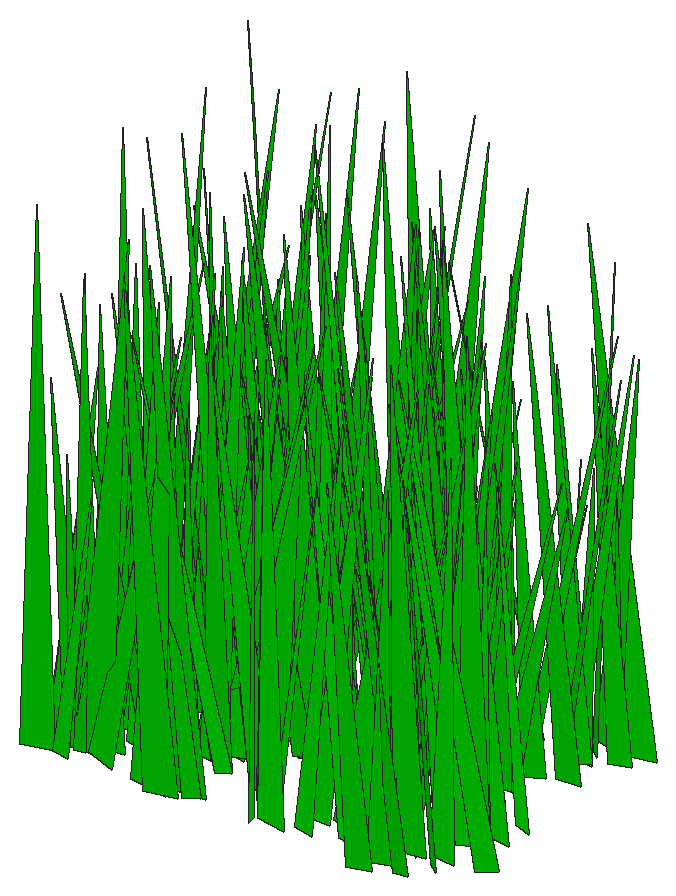
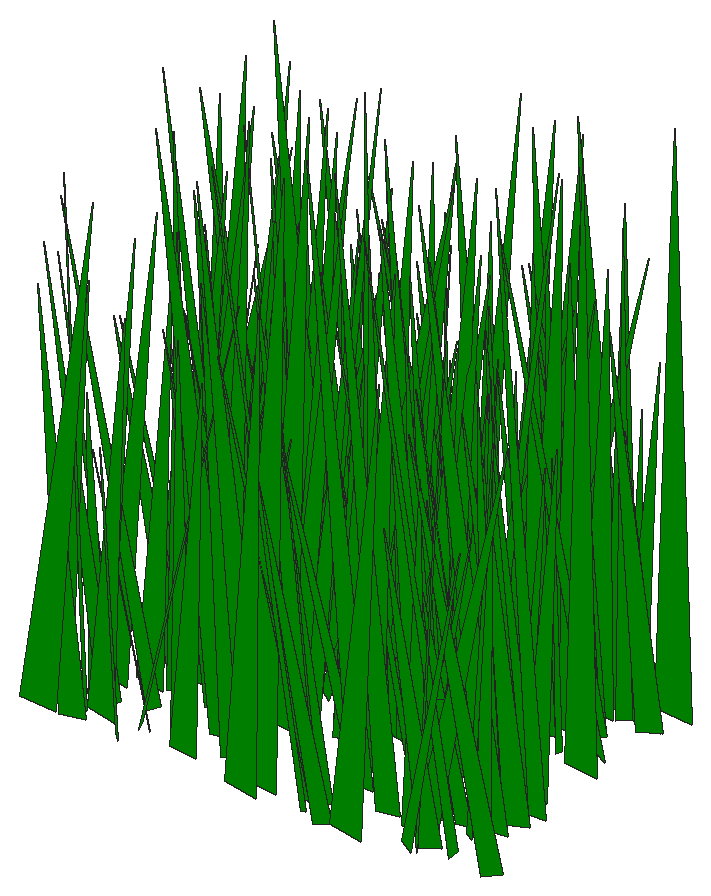
# SketchUp Ruby script. Lengths in inches.
U = 1.inch
M = Sketchup.active_model
def pt(a) = Geom::Point3d.new(a.map { |v| v * U })
def face(e, loops, mat)
  f = e.add_face(loops[0].map { |a| pt(a) })
  loops[1..].each { |l| e.add_face(l.map { |a| pt(a) }).erase! }
  f.material = f.back_material = mat if mat
  f
end
# faces: each face lists its corners as indices into pts; further lists are holes
def faces(e, pts, list, mat = nil) = list.each { |f| face(e, (f[0].is_a?(Array) ? f : [f]).map { |l| l.map { |i| pts[i] } }, mat) }
# xy, xz, yz: faces in a plane at the given z, y or x. An outline is a flat list of corners, or four numbers for a rectangle; further outlines are holes
def ring(l) = l.size == 4 ? [[l[0], l[1]], [l[2], l[1]], [l[2], l[3]], [l[0], l[3]]] : l.each_slice(2).to_a
def flat(e, list, mat, &to3) = list.each { |f| face(e, (f[0].is_a?(Array) ? f : [f]).map { |l| ring(l).map { |u, v| to3.(u, v) } }, mat) }
def xy(e, z, list, mat = nil) = flat(e, list, mat) { |x, y| [x, y, z] }
def xz(e, y, list, mat = nil) = flat(e, list, mat) { |x, z| [x, y, z] }
def yz(e, x, list, mat = nil) = flat(e, list, mat) { |y, z| [x, y, z] }
def lines(e, pts, list) = list.each { |a, b| e.add_line(pt(pts[a]), pt(pts[b])) }
# prism: a flat outline (further loops are holes) pulled along v
def prism(e, loops, v, mat = nil)
  f = face(e, loops, mat); d = Geom::Vector3d.new(v.map { |x| x * U })
  f.pushpull(f.normal.samedirection?(d) ? d.length : -d.length)
end
def box(e, o, s, mat = nil) = prism(e, [[o, [o[0] + s[0], o[1], o[2]], [o[0] + s[0], o[1] + s[1], o[2]], [o[0], o[1] + s[1], o[2]]]], [0, 0, s[2]], mat)
def at(x, y, z, deg = 0) = Geom::Transformation.translation(pt([x, y, z])) * Geom::Transformation.rotation(ORIGIN, Z_AXIS, deg.degrees)
def axes(o, x, y, z) = Geom::Transformation.new([*x, 0, *y, 0, *z, 0, *pt(o).to_a, 1])
def part(name) = M.definitions.add(name)
# library, detail: a bought-in or finely detailed component or shape, given as its bounding box
def library(name, o, s) = part(name).tap { |d| box(d.entities, o, s) }
def detail(e, o, s) = box(e.add_group.entities, o, s)
def put(e, d, t, mat = nil) = e.add_instance(d, t).tap { |i| i.material = mat if mat }
def group(e, t, mat = nil) = e.add_group.tap { |g| g.transformation = t; g.material = mat if mat }.entities
root = M.entities
M.materials.add("[Color G06]").color = [0, 204, 0]
c1 = part("fur_instance\#9")
p = [[0.8125,0,1.79],[0.67,-0.02,1.48],[0,-0.11,0],[0,0.11,0]]
faces(c1.entities,p,[[0,1,2,3]])
put(root,c1,axes([54.39,21.29,4.28],[-0.32887,0.46438,1.72986],[3.51347,0.02974,0.5749],[-0.29205,-0.16513,4.96826]),"[Color G06]")
put(root,c1,axes([54.4,23.9,4.28],[4.17535,-0.0739,3.413],[-0.23891,-0.66047,-0.99003],[-2.33208,-0.06466,6.21204]),"[Color G06]")
put(root,c1,axes([55.41,24.38,4.28],[-3.216,0.412,0.55463],[2.97627,0.4423,0.80624],[-0.09509,-0.09034,6.47707]),"[Color G06]")
put(root,c1,axes([54.22,23.56,4.28],[3.35775,0.35388,2.56454],[2.52243,-0.52084,0.8788],[-1.73834,-0.07222,6.2288]),"[Color G06]")
put(root,c1,axes([52.72,25.09,4.28],[3.14492,-0.38862,0.66664],[-2.81983,-0.42872,1.00531],[0.11909,0.11131,6.19928]),"[Color G06]")
put(root,c1,axes([54.25,15.9,4.28],[2.70284,-0.68709,2.07562],[-4.99876,-0.40147,-0.72645],[-1.10438,0.13558,8.36796]),"[Color G06]")
put(root,c1,axes([53.69,22.07,4.28],[4.95219,0.39046,2.95138],[3.0826,-0.719,-0.62677],[-1.49582,-0.18905,8.47946]),"[Color G06]")
put(root,c1,axes([54.32,19.52,4.28],[3.96209,-0.57788,2.65528],[-4.16866,-0.59516,-0.98497],[-1.71829,0.1114,8.51222]),"[Color G06]")
put(root,c1,axes([54.9,16.7,4.28],[0.16857,0.49558,1.55991],[3.65308,-0.04633,0.80895],[-0.61231,-0.13996,5.25573]),"[Color G06]")
put(root,c1,axes([55.3125,25.28,4.28],[-2.75872,-0.20781,0.94511],[-1.59434,0.37899,-0.8224],[0.28094,0.11013,4.61354]),"[Color G06]")
put(root,c1,axes([54.84,21.24,4.28],[2.06181,0.28515,2.25548],[2.13746,-0.34115,0.59003],[-1.37485,-0.10276,4.29978]),"[Color G06]")
put(root,c1,axes([55.1,25.16,4.28],[-5.73799,-0.08046,2.98882],[-0.8058,0.83989,-0.85823],[1.91905,0.11209,8.57626]),"[Color G06]")
put(root,c1,axes([53.79,22.75,4.28],[0.61886,-0.50723,0.31793],[-3.60857,-0.08115,0.81733],[0.50473,0.04173,5.45369]),"[Color G06]")
put(root,c1,axes([54.17,16.89,4.28],[0.36145,-0.35493,1.94549],[-2.84398,-0.026,0.63535],[0.29127,0.18658,3.78944]),"[Color G06]")
put(root,c1,axes([54.19,16.95,4.28],[-0.4395,0.54622,1.08378],[3.90573,0.07911,-1.04214],[0.78414,-0.08788,5.79824]),"[Color G06]")
put(root,c1,axes([54.52,22.86,4.28],[-1.83901,-0.44209,2.47492],[-3.40475,0.29592,0.42094],[1.09577,0.17753,5.46154]),"[Color G06]")
put(root,c1,axes([54.1,21.81,4.28],[3.61401,-0.17304,1.5239],[-1.34844,-0.5171,0.3982],[-0.87246,0.08243,5.69704]),"[Color G06]")
put(root,c1,axes([54.95,16.67,4.28],[-1.53114,-0.37036,0.85419],[-2.64416,0.22416,0.57766],[0.62379,0.04111,4.54534]),"[Color G06]")
put(root,c1,axes([53.98,22.42,4.28],[2.19139,-0.2507,0.50243],[-1.8224,-0.29307,0.9561],[0.15541,0.09841,4.1271]),"[Color G06]")
put(root,c1,axes([55.09,16.83,4.28],[4.06238,-0.21355,3.19268],[-1.8501,-0.62183,0.48051],[-1.86698,0.15154,6.4708]),"[Color G06]")
put(root,c1,axes([54.04,23.36,4.28],[3.9698,0.60491,1.9926],[4.50643,-0.55462,-0.71321],[-0.53613,-0.18276,8.75945]),"[Color G06]")
put(root,c1,axes([55.6,24.62,4.28],[0.92736,0.51655,0.50005],[3.6541,-0.1355,0.94194],[-0.69385,-0.02321,5.62895]),"[Color G06]")
put(root,c1,axes([54.64,21.84,4.28],[1.4992,0.48907,0.74233],[3.53969,-0.20399,-0.52959],[0.13419,-0.083,5.67598]),"[Color G06]")
put(root,c1,axes([55.26,16.42,4.28],[2.49706,0.29446,1.60599],[2.14462,-0.37344,0.41704],[-1.00716,-0.06513,4.86978]),"[Color G06]")
put(root,c1,axes([54.79,24.99,4.28],[-0.05361,0.4756,0.01399],[3.34161,0.00759,-1.02035],[0.68277,0.00022,4.99493]),"[Color G06]")
put(root,c1,axes([56.28,23.64,4.28],[-2.08549,-0.28281,0.67775],[-2.07819,0.2842,-0.66105],[0.00923,0.08832,4.29725]),"[Color G06]")
put(root,c1,axes([55.39,16.55,4.28],[1.69023,-0.63644,1.78454],[-4.66449,-0.25194,-0.45308],[-0.70656,0.14072,7.26]),"[Color G06]")
put(root,c1,axes([55.33,19.16,4.28],[2.45742,0.11817,1.80132],[1.13854,-0.35975,-0.75845],[-0.93512,-0.12747,3.81028]),"[Color G06]")
put(root,c1,axes([55.16,17.59,4.28],[2.74488,-0.06523,1.24442],[-0.40367,-0.39945,-0.41655],[-0.86554,-0.02058,4.14068]),"[Color G06]")
put(root,c1,axes([54.98,15.96,4.28],[1.92096,-0.27343,1.19339],[-2.10067,-0.26489,0.58119],[-0.26385,0.11826,4.06121]),"[Color G06]")
put(root,c1,axes([54.13,24.88,4.28],[5.77126,-0.07264,1.65356],[-0.6218,-0.81519,0.73366],[-1.05301,0.08323,8.62952]),"[Color G06]")
put(root,c1,axes([55.86,16.97,4.28],[-0.07198,0.64257,1.00658],[4.64555,0.00333,0.49762],[-0.32595,-0.09439,6.86985]),"[Color G06]")
put(root,c1,axes([55.76,18.18,4.28],[0.38893,0.70323,0.41389],[5.03381,-0.05713,0.58507],[-0.41212,-0.03418,7.53692]),"[Color G06]")
put(root,c1,axes([55.11,21.39,4.28],[-2.85975,0.29525,3.99207],[2.87232,0.47051,0.59866],[1.83502,-0.27635,5.28429]),"[Color G06]")
put(root,c1,axes([54.86,23.54,4.28],[1.90639,0.3389,0.36117],[2.44012,-0.26248,-0.47701],[0.10354,-0.05392,4.59177]),"[Color G06]")
put(root,c1,axes([54.96,22.7,4.28],[-2.44366,-0.51435,4.27043],[-4.22034,0.43545,0.6304],[1.98946,0.29197,6.58268]),"[Color G06]")
put(root,c1,axes([56.14,23.07,4.28],[-2.4222,-0.16072,1.56561],[-1.40113,0.3428,-0.79952],[0.68014,0.13382,3.92857]),"[Color G06]")
put(root,c1,axes([56.84,18.28,4.28],[2.06357,-0.41111,4.06457],[-3.41801,-0.4034,-0.81078],[-2.09874,0.25276,5.3169]),"[Color G06]")
put(root,c1,axes([55.32,17.73,4.28],[2.4105,-0.28915,0.19332],[-2.00695,-0.33122,-1.01055],[-0.53712,-0.06004,4.64352]),"[Color G06]")
put(root,c1,axes([57.46,16.8,4.28],[-3.99959,-0.37213,0.86302],[-2.72854,0.55002,-1.00142],[0.10108,0.12253,7.11603]),"[Color G06]")
put(root,c1,axes([54.55,18.6,4.28],[4.47178,0.41149,0.17523],[2.91592,-0.6199,1.00676],[-0.46818,0.06949,7.94392]),"[Color G06]")
put(root,c1,axes([57.03,20.02,4.28],[-5.43427,-0.32024,1.64444],[-2.20505,0.77263,1.00717],[1.2737,-0.02872,8.75967]),"[Color G06]")
put(root,c1,axes([56.06,19.92,4.28],[-1.94851,-0.34259,1.45943],[-2.44364,0.29794,0.74664],[1.00898,0.05999,4.62667]),"[Color G06]")
put(root,c1,axes([56.49,18.41,4.28],[1.89484,-0.65521,2.90311],[-4.94694,-0.30434,-0.67805],[-1.17417,0.22486,7.54167]),"[Color G06]")
put(root,c1,axes([55.21,20.34,4.28],[2.42337,0.26843,0.58382],[1.96182,-0.32647,-0.94651],[0.09764,-0.10286,4.52767]),"[Color G06]")
put(root,c1,axes([55.08,17.96,4.28],[3.47494,-0.38303,1.16165],[-2.84618,-0.47804,0.91113],[-0.22013,0.13428,6.55718]),"[Color G06]")
put(root,c1,axes([55.64,16.5,4.28],[1.06191,-0.77881,1.43715],[-5.65566,-0.13692,0.81096],[0.36184,0.14546,8.45802]),"[Color G06]")
put(root,c1,axes([56.25,20.77,4.28],[-0.48812,-0.56435,0.59145],[-4.0461,0.07295,0.53768],[0.40605,0.04854,6.06878]),"[Color G06]")
put(root,c1,axes([56.42,17.59,4.28],[-0.81081,0.43637,0.59606],[3.1308,0.11836,-0.44094],[0.38738,-0.04321,4.81134]),"[Color G06]")
put(root,c1,axes([55.9,19.44,4.28],[-2.00864,0.36267,2.32372],[2.62384,0.33828,-0.99869],[1.51554,-0.105,4.80878]),"[Color G06]")
put(root,c1,axes([56.95,25.68,4.28],[0.02737,-0.60684,1.90999],[-4.50307,-0.02493,-0.76568],[-0.54191,0.17649,6.45898]),"[Color G06]")
put(root,c1,axes([55.82,23.73,4.28],[2.15587,0.69515,2.44048],[5.24335,-0.29297,-0.76006],[-0.15789,-0.23747,8.08183]),"[Color G06]")
put(root,c1,axes([56.49,17.54,4.28],[-1.58986,0.63127,0.88104],[4.48752,0.23209,-1.01454],[0.83865,-0.04518,7.09892]),"[Color G06]")
put(root,c1,axes([55.61,22.13,4.28],[3.80806,0.03495,0.96703],[0.35187,-0.53107,-0.89046],[-0.59803,-0.08994,5.6338]),"[Color G06]")
put(root,c1,axes([56.38,18.66,4.28],[-0.3077,-0.67019,0.64192],[-4.80571,0.04796,0.60615],[0.43369,0.05593,7.17218]),"[Color G06]")
put(root,c1,axes([56.35,22.41,4.28],[2.4729,0.11645,1.4233],[1.02559,-0.35504,-0.64338],[-0.74329,-0.10245,3.84757]),"[Color G06]")
put(root,c1,axes([56.45,20.07,4.28],[2.32899,-0.5225,0.84399],[-3.72888,-0.33246,-0.65873],[-0.674,0.03384,6.5608]),"[Color G06]")
put(root,c1,axes([57.51,21.8,4.28],[-0.5988,0.63341,0.59432],[4.53264,0.0766,0.82237],[-0.49597,-0.06464,6.798]),"[Color G06]")
put(root,c1,axes([57.01,18.22,4.28],[1.53188,0.34391,1.42378],[2.4933,-0.23899,0.6392],[-0.87952,-0.0785,4.29188]),"[Color G06]")
put(root,c1,axes([56.7,21.53,4.28],[2.75815,-0.30181,0.88619],[-2.08377,-0.39307,-0.89114],[-0.83298,-0.01604,5.16358]),"[Color G06]")
put(root,c1,axes([56.01,16.37,4.28],[2.13686,0.51171,0.80614],[3.69412,-0.28584,-1.02976],[0.33236,-0.11287,6.26251]),"[Color G06]")
put(root,c1,axes([58.96,17.89,4.28],[-3.87655,0.3039,0.26995],[2.18653,0.53782,0.58576],[-0.03539,-0.05997,6.62074]),"[Color G06]")
put(root,c1,axes([57.57,18.24,4.28],[1.99902,0.36205,1.56743],[2.5928,-0.30718,0.76441],[-1.05747,-0.06877,4.83731]),"[Color G06]")
put(root,c1,axes([56.73,24.25,4.28],[4.51231,0.50928,2.87399],[3.98181,-0.64173,-0.90131],[-1.08694,-0.23665,8.62924]),"[Color G06]")
put(root,c1,axes([57.11,21.39,4.28],[2.71803,-0.17288,1.5082],[-1.45728,-0.38206,0.83558],[-0.65701,0.13223,4.38604]),"[Color G06]")
put(root,c1,axes([57.37,20.51,4.28],[3.59461,-0.15483,2.07327],[-1.27584,-0.52874,0.40506],[-1.23671,0.09543,5.60827]),"[Color G06]")
put(root,c1,axes([58.6,18.72,4.28],[-5.08907,0.45043,2.63466],[3.43381,0.7321,0.43775],[1.32304,-0.1675,8.99813]),"[Color G06]")
put(root,c1,axes([57.23,21.55,4.28],[3.53384,-0.42545,1.3267],[-3.03521,-0.50675,-0.60886],[-0.94033,0.03682,6.95111]),"[Color G06]")
put(root,c1,axes([58.39,15.9375,4.28],[0.15133,-0.73593,1.78238],[-5.37361,-0.03986,-0.87169],[-0.63166,0.16282,7.84263]),"[Color G06]")
put(root,c1,axes([57.79,21.41,4.28],[-1.28026,0.55064,0.96088],[3.92353,0.19121,-0.91038],[0.78247,-0.05785,6.13705]),"[Color G06]")
put(root,c1,axes([58.72,22.66,4.28],[-0.92109,0.66321,2.02919],[4.94228,0.11589,0.65999],[-0.19317,-0.19726,7.21021]),"[Color G06]")
put(root,c1,axes([57.92,16.02,4.28],[-0.71518,0.71953,2.07998],[5.30775,0.11849,-0.6322],[0.62412,-0.18321,7.75991]),"[Color G06]")
put(root,c1,axes([58.87,19.34,4.28],[1.63729,0.51899,3.33742],[4.11223,-0.29196,0.70908],[-1.38849,-0.25268,6.03548]),"[Color G06]")
put(root,c1,axes([57.82,18.43,4.28],[2.12451,0.36732,0.0027],[2.61968,-0.29466,0.52674],[-0.27546,0.03066,5.03029]),"[Color G06]")
put(root,c1,axes([59.17,19.12,4.28],[-1.39523,0.73043,1.61988],[5.3465,0.18562,0.6715],[-0.16474,-0.16199,8.07378]),"[Color G06]")
put(root,c1,axes([58.95,16.4,4.28],[-0.78502,-0.76352,1.32542],[-5.54355,0.10374,-0.46905],[-0.18897,0.1285,8.25378]),"[Color G06]")
put(root,c1,axes([59.21,21.04,4.28],[-2.102,0.46139,1.74394],[3.50405,0.28558,0.75485],[0.17569,-0.1756,5.80984]),"[Color G06]")
put(root,c1,axes([57.59,19.98,4.28],[3.03483,-0.40436,0.19445],[-2.88553,-0.42312,-0.47865],[-0.31514,-0.01981,6.25516]),"[Color G06]")
put(root,c1,axes([59.16,16.29,4.28],[0.79739,-0.36655,2.11193],[-2.80611,-0.16152,-0.85385],[-1.01602,0.15843,4.01571]),"[Color G06]")
put(root,c1,axes([58.55,18.16,4.28],[-1.66725,-0.62781,0.91343],[-4.47233,0.24277,0.93339],[0.80081,0.04875,7.11442]),"[Color G06]")
put(root,c1,axes([58.05,25.36,4.28],[3.64071,0.04982,1.4894],[0.55145,-0.51408,-1.03573],[-0.90367,-0.113,5.36844]),"[Color G06]")
put(root,c1,axes([58.73,19.44,4.28],[-2.72797,-0.26611,1.66018],[-1.83308,0.41019,0.8246],[1.23101,0.0211,4.90692]),"[Color G06]")
put(root,c1,axes([57.68,25.69,4.28],[2.12937,-0.36225,0.10794],[-2.58253,-0.29351,0.64819],[0.29009,0.04607,4.97819]),"[Color G06]")
put(root,c1,axes([58.75,22.09,4.28],[3.13847,0.53518,2.17763],[3.87198,-0.47088,0.82874],[-1.36397,-0.10528,7.3633]),"[Color G06]")
put(root,c1,axes([58.37,18.1875,4.28],[3.4486,-0.5114,3.09454],[-4.08796,-0.49621,0.75618],[-1.01266,0.26153,7.48582]),"[Color G06]")
put(root,c1,axes([59.75,20.47,4.28],[-0.95822,-0.82192,0.49987],[-5.87982,0.12862,-0.88245],[-0.5303,0.05904,8.88124]),"[Color G06]")
put(root,c1,axes([58.11,23.62,4.28],[4.30637,0.53799,2.47847],[4.06781,-0.61667,-0.41087],[-1.04289,-0.18383,8.6316]),"[Color G06]")
put(root,c1,axes([60.6,21.05,4.28],[-4.22859,-0.55205,1.16],[-4.03337,0.5818,-1.03581],[0.08462,0.14462,8.59523]),"[Color G06]")
put(root,c1,axes([58.64,21.125,4.28],[1.61668,-0.37402,0.20253],[-2.6598,-0.22604,-0.52636],[-0.37142,-0.00929,4.65093]),"[Color G06]")
put(root,c1,axes([58.18,20.9,4.28],[4.27771,-0.5433,1.48306],[-3.88356,-0.61065,-0.67621],[-1.04048,0.04556,8.62125]),"[Color G06]")
put(root,c1,axes([60.08,19.86,4.28],[-1.87563,-0.47801,0.80167],[-3.46344,0.25286,-0.78083],[-0.20746,0.10032,5.78764]),"[Color G06]")
put(root,c1,axes([58.44,18.8,4.28],[0.79738,0.6295,0.42818],[4.50475,-0.10683,-0.69704],[0.41059,-0.05047,6.81591]),"[Color G06]")
put(root,c1,axes([60.41,17.79,4.28],[-1.9525,0.56587,0.26449],[4.05183,0.26941,0.59929],[-0.28519,-0.04641,6.70376]),"[Color G06]")
put(root,c1,axes([58.21,21.58,4.28],[3.99083,0.17442,0.90425],[1.31098,-0.55769,-0.56671],[-0.46037,-0.07611,6.22495]),"[Color G06]")
put(root,c1,axes([59.91,21.93,4.28],[-1.99997,0.51802,0.05199],[3.69424,0.2779,-0.63818],[0.39239,0.02398,6.27325]),"[Color G06]")
put(root,c1,axes([58.49,24.89,4.28],[2.8164,-0.57635,1.07928],[-4.19556,-0.38799,0.65485],[-0.03924,0.11766,7.44635]),"[Color G06]")
put(root,c1,axes([59.44,21.51,4.28],[5.43606,-0.30262,3.39083],[-2.15748,-0.81962,-0.67683],[-2.28082,0.05405,8.72187]),"[Color G06]")
put(root,c1,axes([60.28,25.16,4.28],[-1.03919,0.84047,2.00881],[6.17195,0.13515,0.63644],[-0.20184,-0.19458,9.11883]),"[Color G06]")
put(root,c1,axes([59.13,19.63,4.28],[1.41917,0.69214,1.86485],[5.11797,-0.19167,-0.52802],[0.00726,-0.18083,7.69757]),"[Color G06]")
put(root,c1,axes([58.32,18.96,4.28],[4.46258,-0.19023,0.98565],[-1.44564,-0.62021,0.86962],[-0.45397,0.10504,6.9199]),"[Color G06]")
put(root,c1,axes([58.29,25.19,4.28],[4.32118,-0.08075,0.51573],[-0.62441,-0.59712,0.94573],[-0.25408,0.09405,6.44706]),"[Color G06]")
put(root,c1,axes([58.45,25.49,4.28],[5.89893,0.16805,1.7197],[1.31074,-0.83244,-0.69855],[-1.0287,-0.09703,8.97133]),"[Color G06]")
put(root,c1,axes([58.25,18.82,4.28],[4.61204,-0.30361,0.7221],[-2.2251,-0.63692,0.9821],[-0.15149,0.11175,7.559]),"[Color G06]")
put(root,c1,axes([60.5,19.87,4.28],[-0.3333,-0.71826,2.44646],[-5.39142,0.0282,-0.68969],[-0.37782,0.23123,7.68346]),"[Color G06]")
put(root,c1,axes([60.38,25.6,4.28],[0.5182,0.61605,2.55432],[4.69726,-0.09778,0.58028],[-0.61144,-0.22904,6.62267]),"[Color G06]")
put(root,c1,axes([58.83,22.92,4.28],[2.83901,-0.2265,0.08443],[-1.61838,-0.3925,0.5972],[0.1498,0.05225,4.8519]),"[Color G06]")
put(root,c1,axes([59.08,21.24,4.28],[3.33968,0.04709,0.53102],[0.36826,-0.46621,-0.42378],[-0.32355,-0.04452,4.99893]),"[Color G06]")
put(root,c1,axes([60.52,21.24,4.28],[-2.41967,0.42221,0.44379],[2.95459,0.33873,-1.03542],[0.72517,0.02866,5.69944]),"[Color G06]")
put(root,c1,axes([59.96,21.49,4.28],[1.80425,-0.33714,0.09973],[-2.3954,-0.25069,-0.54939],[-0.33428,-0.02326,4.47511]),"[Color G06]")
put(root,c1,axes([61.76,20.49,4.28],[-2.52677,-0.20544,0.08317],[-1.44438,0.34187,-1.01526],[-0.29545,0.08565,4.25194]),"[Color G06]")
put(root,c1,axes([60.96,24.43,4.28],[-2.81039,-0.05218,1.15097],[-0.29086,0.40475,0.52161],[0.80529,-0.03592,4.20517]),"[Color G06]")
put(root,c1,axes([60.38,17.51,4.28],[-3.45015,-0.08761,2.55465],[-0.39191,0.53437,0.92286],[1.77842,-0.0522,5.15941]),"[Color G06]")
put(root,c1,axes([61.32,22.36,4.28],[-4.00504,-0.56962,1.14358],[-4.02804,0.56852,1.01923],[1.02315,0.00848,8.4891]),"[Color G06]")
put(root,c1,axes([61.39,21.5625,4.28],[-3.6716,-0.46883,1.08752],[-3.30746,0.52192,0.90403],[0.9455,0.00515,7.38546]),"[Color G06]")
put(root,c1,axes([61.98,20.65,4.28],[-5.84338,0.22169,2.4058],[1.73347,0.8382,0.53209],[1.45384,-0.10839,9.03516]),"[Color G06]")
put(root,c1,axes([60.13,20.59,4.28],[3.55356,-0.32669,0.74331],[-2.32802,-0.50031,-0.39914],[-0.5624,0.00679,6.34887]),"[Color G06]")
put(root,c1,axes([61.18,23.95,4.28],[-1.78136,-0.58122,0.73063],[-4.13485,0.25574,0.85139],[0.71745,0.03079,6.72085]),"[Color G06]")
put(root,c1,axes([61.86,23.96,4.28],[-2.79685,-0.27858,0.15964],[-1.95556,0.38608,0.86498],[0.42223,-0.05717,5.06361]),"[Color G06]")
put(root,c1,axes([60.45,24.89,4.28],[3.31748,0.70859,0.79572],[5.0628,-0.46782,0.7067],[-0.68762,-0.02579,9.04228]),"[Color G06]")
put(root,c1,axes([61.12,16.36,4.28],[3.80722,-0.0541,2.40725],[-0.27598,-0.57573,-0.51143],[-1.63358,-0.02883,5.69672]),"[Color G06]")
put(root,c1,axes([61.69,22.4375,4.28],[-3.10528,0.64494,3.57247],[5.13043,0.44506,0.73147],[0.88509,-0.31705,8.29381]),"[Color G06]")
put(root,c1,axes([60.88,20.4,4.28],[2.66209,0.15886,1.53407],[1.33513,-0.38116,-0.64103],[-0.7542,-0.11403,4.27997]),"[Color G06]")
put(root,c1,axes([61.68,16.49,4.28],[-2.98952,0.50876,1.5907],[3.63189,0.43806,-0.84772],[1.11942,-0.06257,6.99846]),"[Color G06]")
put(root,c1,axes([62.11,21.24,4.28],[-3.19544,-0.26028,1.77902],[-2.0705,0.45453,-0.66803],[0.78348,0.13964,5.4904]),"[Color G06]")
put(root,c1,axes([62.78,20.29,4.28],[-2.78088,-0.4483,0.42594],[-3.22742,0.38587,-0.41342],[-0.02363,0.05528,6.3396]),"[Color G06]")
put(root,c1,axes([61.39,22.02,4.28],[4.04129,0.41683,3.02844],[3.36318,-0.58888,-0.71408],[-1.31537,-0.22502,7.4787]),"[Color G06]")
put(root,c1,axes([61.44,24.4375,4.28],[-1.1828,0.57646,2.42323],[4.29957,0.20716,-0.97336],[1.11003,-0.18816,6.3523]),"[Color G06]")
put(root,c1,axes([61.25,17.28,4.28],[3.42408,-0.13027,1.02892],[-0.89207,-0.48677,-0.44848],[-0.74224,-0.01594,5.28561]),"[Color G06]")
put(root,c1,axes([62.125,21.31,4.28],[1.08917,0.4069,1.09825],[2.9541,-0.16532,0.49217],[-0.57251,-0.07896,4.62892]),"[Color G06]")
put(root,c1,axes([63.09,20.03,4.28],[-1.32728,0.40622,0.55017],[2.89561,0.17174,1.0377],[-0.48699,-0.08601,4.67059]),"[Color G06]")
put(root,c1,axes([61.61,18.46,4.28],[-0.25455,-0.53455,1.85389],[-3.96706,0.06355,0.8882],[0.70431,0.16474,5.67281]),"[Color G06]")
put(root,c1,axes([61.52,21.6875,4.28],[5.44106,-0.04713,2.26202],[-0.48751,-0.78293,0.74532],[-1.47215,0.08506,8.11357]),"[Color G06]")
put(root,c1,axes([62.7,25.01,4.28],[0.63302,-0.49858,1.20645],[-3.62789,-0.10153,-0.56774],[-0.52314,0.10077,5.39706]),"[Color G06]")
put(root,c1,axes([63.21,22.85,4.28],[-3.41123,0.02386,1.13545],[0.10236,0.4856,-0.48517],[0.77198,0.04103,5.08164]),"[Color G06]")
put(root,c1,axes([62.9375,19.84,4.28],[-2.66429,-0.65679,1.33858],[-4.72583,0.38384,0.62425],[0.80814,0.07931,8.06354]),"[Color G06]")
put(root,c1,axes([62.87,23.06,4.28],[-3.62473,-0.61461,2.50056],[-4.52135,0.53656,0.50973],[1.33532,0.14839,8.51367]),"[Color G06]")
put(root,c1,axes([62.9,22.33,4.28],[2.75165,0.00009,2.16847],[-0.26379,-0.42652,0.74985],[-1.42672,0.07904,4.0436]),"[Color G06]")
put(root,c1,axes([64.38,24.58,4.28],[-4.81775,0.01951,0.519],[0.09704,0.66872,-0.8762],[0.3616,0.08053,7.15003]),"[Color G06]")
put(root,c1,axes([62.5,23.16,4.28],[2.59938,-0.01504,1.17064],[-0.21911,-0.37433,0.53437],[-0.75969,0.05651,3.85141]),"[Color G06]")
put(root,c1,axes([63.76,21.94,4.28],[-4.44107,-0.39345,2.4379],[-3.07817,0.63269,-0.79571],[1.07083,0.18696,7.82346]),"[Color G06]")
put(root,c1,axes([63.93,17,4.28],[-3.71389,0.41063,0.56553],[2.89565,0.51964,-0.86622],[0.65551,0.03099,7.03059]),"[Color G06]")
put(root,c1,axes([63.6,18.09,4.28],[-0.34919,-0.40769,1.31458],[-3.01797,0.02742,-0.81367],[-0.46167,0.12908,4.32476]),"[Color G06]")
put(root,c1,axes([62.58,16.74,4.28],[3.27232,-0.26433,1.99585],[-2.14726,-0.46701,0.75886],[-0.87514,0.15747,5.60088]),"[Color G06]")
put(root,c1,axes([63.04,17.86,4.28],[-2.03946,-0.32178,1.99351],[-2.42149,0.32156,0.42884],[1.11377,0.10989,4.58277]),"[Color G06]")
put(root,c1,axes([61.92,23.72,4.28],[3.90134,-0.12561,0.27688],[-0.86648,-0.53979,-0.85957],[-0.30816,-0.07248,5.9222]),"[Color G06]")
put(root,c1,axes([62.27,23.76,4.28],[2.58214,0.72752,1.71972],[5.34254,-0.35233,-0.79622],[-0.02155,-0.17679,8.66374]),"[Color G06]")
put(root,c1,axes([63.23,24.4,4.28],[-1.70467,-0.44282,1.99354],[-3.32864,0.26514,0.40749],[0.88521,0.14424,5.3713]),"[Color G06]")
put(root,c1,axes([62.59,19.55,4.28],[2.58148,-0.77152,1.99134],[-5.68827,-0.35604,0.62547],[-0.17387,0.19323,9.10345]),"[Color G06]")
put(root,c1,axes([62.54,17.4375,4.28],[4.05306,-0.40822,1.71043],[-3.04839,-0.57398,0.39888],[-0.76611,0.12426,7.46179]),"[Color G06]")
put(root,c1,axes([63.69,22.03,4.28],[-1.11822,-0.41786,0.61917],[-2.99548,0.16155,0.43988],[0.42227,0.03943,4.76002]),"[Color G06]")
put(root,c1,axes([64.34,21.48,4.28],[-0.58697,-0.41103,0.23924],[-2.90407,0.07632,-0.85256],[-0.52955,0.03705,4.41028]),"[Color G06]")
put(root,c1,axes([63.2,21.86,4.28],[3.86295,0.32702,1.5601],[2.30744,-0.5576,0.66438],[-1.12472,-0.02079,6.72133]),"[Color G06]")
put(root,c1,axes([64.43,18.13,4.28],[-3.07439,0.12255,0.98117],[0.7654,0.43479,-0.88125],[0.78582,0.05597,4.697]),"[Color G06]")
put(root,c1,axes([63.53,18.09,4.28],[0.90235,-0.36214,0.39562],[-2.60086,-0.12137,0.4884],[0.22385,0.04964,4.07992]),"[Color G06]")
put(root,c1,axes([63,21.69,4.28],[3.70436,0.00302,0.65947],[-0.03105,-0.51652,0.66143],[-0.44068,0.06179,5.49688]),"[Color G06]")
put(root,c1,axes([64.61,18.49,4.28],[0.31204,0.4639,0.47436],[3.28929,-0.05049,0.83862],[-0.59039,-0.0361,4.92298]),"[Color G06]")
put(root,c1,axes([65.11,21.4,4.28],[-4.34918,-0.02184,1.42835],[-0.03876,0.61658,0.81933],[0.96766,-0.07346,6.45257]),"[Color G06]")
put(root,c1,axes([64.36,19.15,4.28],[2.41986,-0.35044,1.93911],[-2.55864,-0.37272,-0.60554],[-1.20521,0.08763,5.17895]),"[Color G06]")
put(root,c1,axes([64.66,18.04,4.28],[-3.29788,-0.54686,1.50326],[-3.90744,0.47728,0.79709],[1.05981,0.05798,7.61663]),"[Color G06]")
put(root,c1,axes([63.46,22.73,4.28],[1.75399,-0.40834,0.5947],[-2.95101,-0.23856,0.62468],[0.15807,0.07739,5.06325]),"[Color G06]")
put(root,c1,axes([65.37,21.04,4.28],[-3.05703,0.6537,2.08462],[4.88057,0.42264,0.76283],[0.31811,-0.2023,8.32956]),"[Color G06]")
put(root,c1,axes([64.86,22.07,4.28],[-3.39765,-0.08178,1.4692],[-0.43979,0.48966,0.85904],[1.0568,-0.05914,5.08101]),"[Color G06]")
put(root,c1,axes([63.49,17.57,4.28],[1.14283,0.69555,0.25658],[4.96001,-0.15555,-0.9083],[0.55465,-0.04211,7.59393]),"[Color G06]")
put(root,c1,axes([64.26,18.35,4.28],[-0.21511,0.37782,0.46166],[2.69984,0.03559,-0.53573],[0.38386,-0.03858,4.02671]),"[Color G06]")
put(root,c1,axes([65,16.08,4.28],[-0.18633,-0.55422,1.11895],[-4.02383,0.01488,-0.64989],[-0.40713,0.10655,5.91105]),"[Color G06]")
put(root,c1,axes([63.7,19.11,4.28],[2.51787,0.26663,0.78198],[1.978,-0.34573,-0.68462],[-0.13148,-0.09522,4.67538]),"[Color G06]")
put(root,c1,axes([65.36,19.23,4.28],[-4.91467,0.33135,2.84236],[2.68405,0.70933,0.86765],[1.43487,-0.19196,8.11254]),"[Color G06]")
put(root,c1,axes([64.47,25.42,4.28],[2.62273,0.0989,1.2956],[0.59501,-0.3838,0.67487],[-0.9489,0.03269,4.00418]),"[Color G06]")
put(root,c1,axes([65.99,19.5,4.28],[-4.15321,-0.20205,0.5205],[-1.417,0.57996,0.60602],[0.46141,-0.03762,6.5462]),"[Color G06]")
put(root,c1,axes([65.32,17.39,4.28],[-2.43532,-0.23615,0.23195],[-1.6206,0.33373,1.0234],[0.51544,-0.06648,4.31356]),"[Color G06]")
put(root,c1,axes([64.19,19.37,4.28],[2.68325,-0.0681,0.86709],[-0.5609,-0.37842,0.46317],[-0.51036,0.05786,4.0498]),"[Color G06]")
put(root,c1,axes([64.73,22.67,4.28],[-2.6046,-0.47414,2.04592],[-3.43245,0.39766,0.82544],[1.28578,0.1011,6.34797]),"[Color G06]")
put(root,c1,axes([64.88,17.42,4.28],[0.59758,0.40369,0.22093],[2.88198,-0.085,0.42871],[-0.31102,-0.012,4.39707]),"[Color G06]")
put(root,c1,axes([65.68,17.62,4.28],[-2.79908,-0.03531,0.59968],[-0.19991,0.3914,0.56279],[0.43027,-0.04783,4.16264]),"[Color G06]")
put(root,c1,axes([64.17,24.52,4.28],[2.69324,0.09883,0.25732],[0.65725,-0.36869,0.90016],[-0.31613,0.07541,4.06378]),"[Color G06]")
put(root,c1,axes([66.02,16.53,4.28],[-4.22483,-0.35814,1.7815],[-2.72939,0.59457,-0.72763],[0.75344,0.1456,7.35364]),"[Color G06]")
put(root,c1,axes([66.12,19.68,4.28],[-2.86896,0.04404,0.15599],[0.29768,0.39635,-0.6238],[0.14835,0.05631,4.26842]),"[Color G06]")
put(root,c1,axes([66.42,18.81,4.28],[-3.56805,0.35022,0.60367],[2.53862,0.49643,0.43233],[0.16235,-0.06547,6.507]),"[Color G06]")
put(root,c1,axes([65.49,24.8,4.28],[1.11275,-0.51072,1.68047],[-3.73605,-0.18082,-0.78667],[-0.84865,0.12636,5.66663]),"[Color G06]")
put(root,c1,axes([63.65,19.76,4.28],[2.60056,-0.70347,0.06316],[-5.01525,-0.35977,0.95102],[0.54636,0.04586,8.42911]),"[Color G06]")
put(root,c1,axes([65.52,22.8,4.28],[1.79726,-0.48283,1.92331],[-3.51524,-0.28487,-0.8775],[-1.13483,0.11774,5.76413]),"[Color G06]")
put(root,c1,axes([65.1875,21.8,4.28],[3.4223,0.52447,2.4532],[3.84138,-0.51428,0.65996],[-1.44369,-0.12511,7.57136]),"[Color G06]")
put(root,c1,axes([65.52,17.54,4.28],[0.38039,-0.68994,1.86223],[-5.08658,-0.06491,-0.44172],[-0.39917,0.16967,7.40342]),"[Color G06]")
put(root,c1,axes([65.99,19.66,4.28],[-1.18509,0.7917,1.97641],[5.82679,0.15518,0.66378],[-0.1765,-0.19296,8.64286]),"[Color G06]")
put(root,c1,axes([64.82,21.01,4.28],[2.45618,0.3456,0.03456],[2.43973,-0.33793,0.88517],[-0.43672,0.05588,5.13936]),"[Color G06]")
put(root,c1,axes([65.21,16.64,4.28],[2.11225,-0.47648,1.10979],[-3.43229,-0.30564,-0.48205],[-0.66817,0.06374,5.9845]),"[Color G06]")
put(root,c1,axes([66.02,24.19,4.28],[-3.51601,0.35375,2.52542],[2.87807,0.50374,0.84485],[1.00362,-0.2053,6.42461]),"[Color G06]")
put(root,c1,axes([64.63,20.63,4.28],[4.72564,0.48084,1.27584],[3.37875,-0.66957,1.03373],[-1.09676,0.00906,8.68184]),"[Color G06]")
put(root,c1,axes([65.25,18.93,4.28],[3.73599,0.02411,1.82151],[-0.04662,-0.53992,1.03447],[-1.23007,0.09368,5.49313]),"[Color G06]")
put(root,c1,axes([65.01,20.07,4.28],[-1.3903,0.47318,3.54102],[3.89755,0.26691,-0.67899],[1.39183,-0.27477,5.43854]),"[Color G06]")
put(root,c1,axes([66.39,23.18,4.28],[-2.28702,-0.55533,1.9052],[-4.16953,0.31817,-0.52644],[0.31596,0.17908,6.84348]),"[Color G06]")
put(root,c1,axes([64.57,22,4.28],[2.97899,0.27416,0.3146],[1.97719,-0.41239,-0.53665],[0.02334,-0.05795,5.30752]),"[Color G06]")
put(root,c1,axes([67.07,25.34,4.28],[-2.28766,0.70154,0.68756],[5.05031,0.31581,0.51835],[-0.12675,-0.07837,8.24365]),"[Color G06]")
put(root,c1,axes([66.52,17.32,4.28],[-3.64297,-0.16196,1.60866],[-1.10677,0.52969,0.52741],[1.13246,-0.00331,5.69031]),"[Color G06]")
put(root,c1,axes([65.95,24.29,4.28],[-0.82196,0.41173,0.88879],[2.969,0.12522,-0.53035],[0.50664,-0.06583,4.54991]),"[Color G06]")
put(root,c1,axes([66.85,19.55,4.28],[-3.2686,0.51227,0.57031],[3.6397,0.45883,-0.74803],[0.62737,0.00699,7.31099]),"[Color G06]")
put(root,c1,axes([64.63,23.74,4.28],[4.65456,-0.19483,0.93686],[-1.46389,-0.64821,0.76025],[-0.44962,0.09349,7.22335]),"[Color G06]")
put(root,c1,axes([66.19,19.42,4.28],[-1.84932,0.56157,4.1098],[4.8083,0.27832,0.46431],[0.81245,-0.36888,6.60693]),"[Color G06]")
put(root,c1,axes([67.73,18.06,4.28],[-3.74937,0.44948,0.7362],[3.26049,0.5155,0.93739],[-0.04039,-0.11107,7.33015]),"[Color G06]")
put(root,c1,axes([65.96,24.84,4.28],[4.75552,0.12485,2.74298],[1.0574,-0.70545,-0.40633],[-1.74696,-0.08712,7.22093]),"[Color G06]")
put(root,c1,axes([66.91,24.73,4.28],[1.97744,-0.43439,3.03942],[-3.42627,-0.33777,-0.56607],[-1.44925,0.20583,5.48547]),"[Color G06]")
put(root,c1,axes([65.32,21.9,4.28],[1.66831,-0.42516,0.31939],[-3.01488,-0.22333,1.02512],[0.50228,0.07163,5.09229]),"[Color G06]")
put(root,c1,axes([67.04,20.4375,4.28],[-3.30528,0.24006,0.91077],[1.61835,0.46645,-1.00415],[0.84609,0.04559,5.4786]),"[Color G06]")
put(root,c1,axes([66.49,19.45,4.28],[-2.52725,0.28078,1.42335],[1.93061,0.3763,-0.87029],[1.11093,-0.01519,4.75039]),"[Color G06]")
put(root,c1,axes([66.59,25.04,4.28],[1.79093,0.27234,0.97594],[1.83617,-0.26582,0.99467],[-0.93236,-0.00036,3.8335]),"[Color G06]")
put(root,c1,axes([65.99,25.33,4.28],[-0.62251,-0.50211,2.94236],[-4.01171,0.13296,0.71046],[0.8646,0.25539,5.41504]),"[Color G06]")
put(root,c1,axes([66.41,17.8125,4.28],[-2.14151,0.45546,2.18792],[3.40731,0.33226,-0.49574],[1.09601,-0.14301,5.81618]),"[Color G06]")
put(root,c1,axes([65.54,24.07,4.28],[4.03518,0.15816,1.40619],[1.28445,-0.56496,-0.93352],[-0.72242,-0.12104,6.19464]),"[Color G06]")
put(root,c1,axes([65.58,24.44,4.28],[3.89481,-0.26121,1.64563],[-2.06666,-0.54264,1.03147],[-0.67087,0.15519,6.37643]),"[Color G06]")
